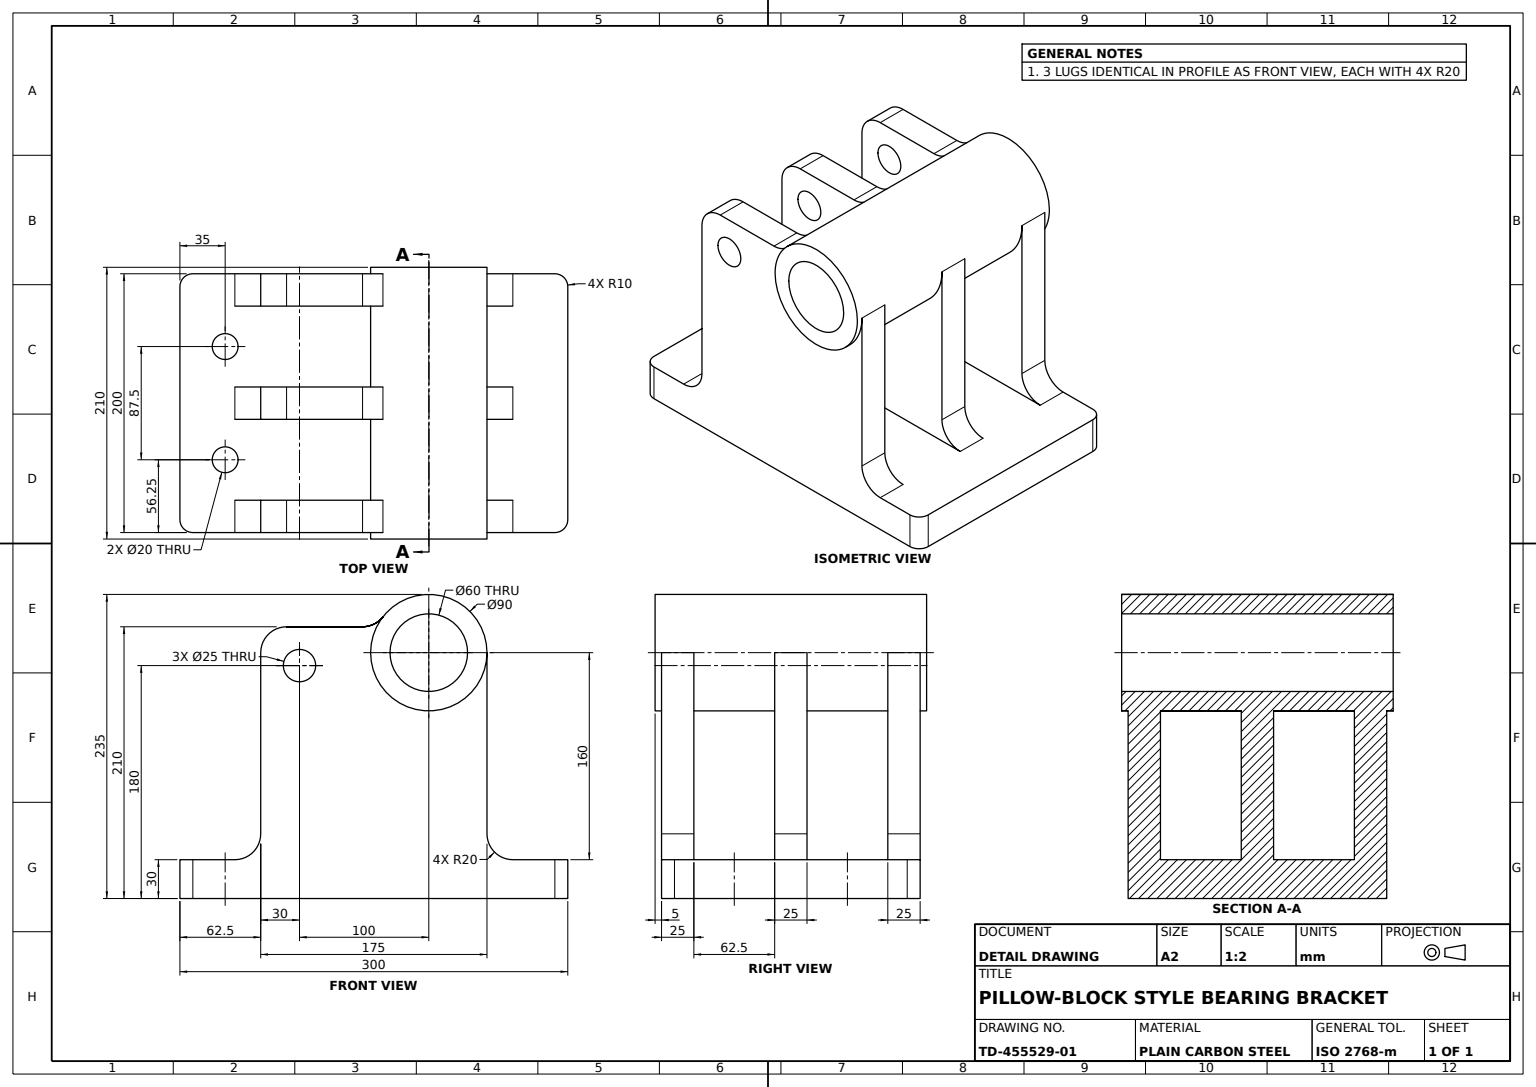
solid
v1 (12.5,50,-87.5)
v2 (-12.5,50,-87.5)
e1 v1 v2 LINE
v3 (12.5,30,-107.5)
e2 v3 v1 CIRCLE(AX(P(12.5,50,-107.5),D(-1,0,0),D(0,0,-1)),20)
v4 (-12.5,30,-107.5)
e3 v4 v3 LINE
e4 v2 v4 CIRCLE(AX(P(-12.5,50,-107.5),D(1,0,0),D(0,0,-1)),20)
face CYL(AX(P(12.5,50,-107.5),D(1,0,0),D(0,0,-1)),20) rev [-e1 -e2 -e3 -e4]
v5 (-75,50,87.5)
v6 (-75,30,107.5)
e5 v5 v6 CIRCLE(AX(P(-75,50,107.5),D(-1,0,0),D(0,0,-1)),20)
v7 (-75,30,-107.5)
e6 v6 v7 LINE
v8 (-75,50,-87.5)
e7 v7 v8 CIRCLE(AX(P(-75,50,-107.5),D(-1,0,0),D(0,0,-1)),20)
v9 (-75,190,-87.5)
e8 v8 v9 LINE
v10 (-75,190,2.5)
e9 v10 v9 CIRCLE(AX(P(-75,190,-42.5),D(1,0,0),D(0,0,-1)),45)
v11 (-75,217.692308,-7.029786)
e10 v11 v10 CIRCLE(AX(P(-75,190,-42.5),D(1,0,0),D(0,0,-1)),45)
v12 (-75,210,8.734754)
e11 v11 v12 CIRCLE(AX(P(-75,230,8.734754),D(-1,0,0),D(0,0,-1)),20)
v13 (-75,210,67.5)
e12 v12 v13 LINE
v14 (-75,190,87.5)
e13 v13 v14 CIRCLE(AX(P(-75,190,67.5),D(1,0,0),D(0,0,-1)),20)
e14 v14 v5 LINE
v15 (-75,180,70)
v16 (-75,180,45)
e15 v15 v16 CIRCLE(AX(P(-75,180,57.5),D(1,0,0),D(0,0,-1)),12.5)
e16 v16 v15 CIRCLE(AX(P(-75,180,57.5),D(1,0,0),D(0,0,-1)),12.5)
face PLANE(AX(P(-75,0,0),D(1,0,0),D(0,0,-1))) [e5 e6 e7 e8 -e9 -e10 e11 e12 e13 e14] [-e15 -e16]
v17 (-12.5,217.692308,-7.029786)
v18 (12.5,217.692308,-7.029786)
e17 v17 v18 LINE
v19 (-12.5,210,8.734754)
e18 v19 v17 CIRCLE(AX(P(-12.5,230,8.734754),D(1,0,0),D(0,0,-1)),20)
v20 (12.5,210,8.734754)
e19 v20 v19 LINE
e20 v18 v20 CIRCLE(AX(P(12.5,230,8.734754),D(-1,0,0),D(0,0,-1)),20)
face CYL(AX(P(-105,230,8.734754),D(1,0,0),D(0,0,-1)),20) rev [-e17 -e18 -e19 -e20]
v21 (-100,180,70)
e21 v21 v15 LINE
v22 (-100,180,45)
e22 v22 v21 CIRCLE(AX(P(-100,180,57.5),D(1,0,0),D(0,0,-1)),12.5)
e23 v22 v16 LINE
face CYL(AX(P(-100,180,57.5),D(1,0,0),D(0,0,-1)),12.5) rev [e16 -e21 -e22 e23]
v23 (-43.75,30,125)
v24 (-43.75,30,105)
e24 v23 v24 CIRCLE(AX(P(-43.75,30,115),D(0,1,0),D(0,0,1)),10)
v25 (-43.75,0,105)
e25 v25 v24 LINE
v26 (-43.75,0,125)
e26 v25 v26 CIRCLE(AX(P(-43.75,0,115),D(0,-1,0),D(0,0,-1)),10)
e27 v26 v23 LINE
face CYL(AX(P(-43.75,-10,115),D(0,1,0),D(0,0,1)),10) rev [e24 -e25 e26 e27]
v27 (43.75,0,105)
v28 (43.75,30,105)
e28 v27 v28 LINE
v29 (43.75,0,125)
e29 v27 v29 CIRCLE(AX(P(43.75,0,115),D(0,-1,0),D(0,0,-1)),10)
v30 (43.75,30,125)
e30 v29 v30 LINE
e31 v30 v28 CIRCLE(AX(P(43.75,30,115),D(0,1,0),D(0,0,1)),10)
face CYL(AX(P(43.75,-10,115),D(0,1,0),D(0,0,1)),10) rev [-e28 e29 e30 e31]
v31 (12.5,190,2.5)
v32 (75,190,2.5)
e32 v31 v32 LINE
v33 (12.5,190,-87.5)
e33 v31 v33 CIRCLE(AX(P(12.5,190,-42.5),D(1,0,0),D(0,0,-1)),45)
v34 (75,190,-87.5)
e34 v33 v34 LINE
e35 v34 v32 CIRCLE(AX(P(75,190,-42.5),D(-1,0,0),D(0,0,1)),45)
face CYL(AX(P(-105,190,-42.5),D(1,0,0),D(0,0,-1)),45) [-e32 e33 e34 e35]
v35 (75,180,45)
v36 (75,180,70)
e36 v35 v36 CIRCLE(AX(P(75,180,57.5),D(-1,0,0),D(0,0,1)),12.5)
e37 v36 v35 CIRCLE(AX(P(75,180,57.5),D(-1,0,0),D(0,0,1)),12.5)
v37 (75,50,-87.5)
e38 v37 v34 LINE
v38 (75,30,-107.5)
e39 v37 v38 CIRCLE(AX(P(75,50,-107.5),D(1,0,0),D(0,0,1)),20)
v39 (75,30,107.5)
e40 v39 v38 LINE
v40 (75,50,87.5)
e41 v39 v40 CIRCLE(AX(P(75,50,107.5),D(1,0,0),D(0,0,1)),20)
v41 (75,190,87.5)
e42 v41 v40 LINE
v42 (75,210,67.5)
e43 v41 v42 CIRCLE(AX(P(75,190,67.5),D(-1,0,0),D(0,0,1)),20)
v43 (75,210,8.734754)
e44 v43 v42 LINE
v44 (75,217.692308,-7.029786)
e45 v43 v44 CIRCLE(AX(P(75,230,8.734754),D(1,0,0),D(0,0,1)),20)
e46 v32 v44 CIRCLE(AX(P(75,190,-42.5),D(-1,0,0),D(0,0,1)),45)
face PLANE(AX(P(75,0,0),D(-1,0,0),D(0,0,1))) [-e36 -e37] [-e38 e39 -e40 e41 -e42 e43 -e44 e45 -e46 -e35]
v45 (100,180,45)
e47 v35 v45 LINE
v46 (100,180,70)
e48 v36 v46 LINE
e49 v46 v45 CIRCLE(AX(P(100,180,57.5),D(1,0,0),D(0,0,-1)),12.5)
face CYL(AX(P(-100,180,57.5),D(1,0,0),D(0,0,-1)),12.5) rev [-e47 e36 e48 e49]
v47 (-100,210,8.734754)
e50 v12 v47 LINE
v48 (-100,210,67.5)
e51 v47 v48 LINE
e52 v48 v13 LINE
face PLANE(AX(P(-65,210,0),D(0,-1,0),D(0,0,-1))) rev [-e12 e50 e51 e52]
v49 (105,190,2.5)
v50 (105,190,-87.5)
e53 v49 v50 CIRCLE(AX(P(105,190,-42.5),D(1,0,0),D(0,0,-1)),45)
v51 (100,190,2.5)
e54 v51 v49 LINE
v52 (100,190,-87.5)
e55 v51 v52 CIRCLE(AX(P(100,190,-42.5),D(1,0,0),D(0,0,-1)),45)
e56 v52 v50 LINE
face CYL(AX(P(-105,190,-42.5),D(1,0,0),D(0,0,-1)),45) [-e53 -e54 e55 e56]
v53 (-100,50,-87.5)
v54 (-100,30,-107.5)
e57 v53 v54 CIRCLE(AX(P(-100,50,-107.5),D(1,0,0),D(0,0,-1)),20)
e58 v8 v53 LINE
e59 v54 v7 LINE
face CYL(AX(P(-65,50,-107.5),D(1,0,0),D(0,0,-1)),20) rev [-e57 -e58 -e7 -e59]
v55 (-100,190,87.5)
e60 v14 v55 LINE
e61 v55 v48 CIRCLE(AX(P(-100,190,67.5),D(-1,0,0),D(0,0,-1)),20)
face CYL(AX(P(-65,190,67.5),D(1,0,0),D(0,0,-1)),20) [-e60 -e13 -e52 -e61]
e62 v21 v22 CIRCLE(AX(P(-100,180,57.5),D(1,0,0),D(0,0,-1)),12.5)
face CYL(AX(P(-100,180,57.5),D(1,0,0),D(0,0,-1)),12.5) rev [e21 e15 -e23 -e62]
e63 v34 v52 LINE
v56 (100,50,-87.5)
e64 v56 v52 LINE
e65 v56 v37 LINE
face PLANE(AX(P(75,30,-87.5),D(0,0,-1),D(-1,0,0))) [e38 e63 -e64 e65]
v57 (-105,190,2.5)
v58 (-100,190,2.5)
e66 v57 v58 LINE
v59 (-105,190,-87.5)
e67 v57 v59 CIRCLE(AX(P(-105,190,-42.5),D(1,0,0),D(0,0,-1)),45)
v60 (-100,190,-87.5)
e68 v59 v60 LINE
e69 v58 v60 CIRCLE(AX(P(-100,190,-42.5),D(1,0,0),D(0,0,-1)),45)
face CYL(AX(P(-105,190,-42.5),D(1,0,0),D(0,0,-1)),45) [-e66 e67 e68 -e69]
e70 v28 v30 CIRCLE(AX(P(43.75,30,115),D(0,1,0),D(0,0,1)),10)
e71 v29 v27 CIRCLE(AX(P(43.75,0,115),D(0,-1,0),D(0,0,-1)),10)
face CYL(AX(P(43.75,-10,115),D(0,1,0),D(0,0,1)),10) rev [e28 e70 -e30 e71]
v61 (-105,190,-72.5)
v62 (-105,190,-12.5)
e72 v61 v62 CIRCLE(AX(P(-105,190,-42.5),D(1,0,0),D(0,0,-1)),30)
e73 v62 v61 CIRCLE(AX(P(-105,190,-42.5),D(1,0,0),D(0,0,-1)),30)
e74 v59 v57 CIRCLE(AX(P(-105,190,-42.5),D(1,0,0),D(0,0,-1)),45)
face PLANE(AX(P(-105,190,-42.5),D(1,0,0),D(0,0,-1))) rev [e72 e73] [-e74 -e67]
e75 v45 v46 CIRCLE(AX(P(100,180,57.5),D(1,0,0),D(0,0,-1)),12.5)
v63 (100,217.692308,-7.029786)
v64 (100,210,8.734754)
e76 v63 v64 CIRCLE(AX(P(100,230,8.734754),D(-1,0,0),D(0,0,1)),20)
v65 (100,210,67.5)
e77 v64 v65 LINE
v66 (100,190,87.5)
e78 v65 v66 CIRCLE(AX(P(100,190,67.5),D(1,0,0),D(0,0,1)),20)
v67 (100,50,87.5)
e79 v66 v67 LINE
v68 (100,30,107.5)
e80 v67 v68 CIRCLE(AX(P(100,50,107.5),D(-1,0,0),D(0,0,1)),20)
v69 (100,30,140)
e81 v69 v68 LINE
v70 (100,0,140)
e82 v69 v70 LINE
v71 (100,0,-140)
e83 v70 v71 LINE
v72 (100,30,-140)
e84 v72 v71 LINE
v73 (100,30,-107.5)
e85 v73 v72 LINE
e86 v73 v56 CIRCLE(AX(P(100,50,-107.5),D(-1,0,0),D(0,0,1)),20)
e87 v63 v51 CIRCLE(AX(P(100,190,-42.5),D(1,0,0),D(0,0,-1)),45)
face PLANE(AX(P(100,30,140),D(-1,0,0),D(0,0,1))) rev [-e75 -e49] [e76 e77 e78 e79 e80 -e81 e82 e83 -e84 -e85 e86 e64 -e55 -e87]
v74 (-100,30,140)
v75 (-100,0,140)
e88 v74 v75 LINE
v76 (-90,0,150)
e89 v75 v76 CIRCLE(AX(P(-90,0,140),D(0,1,0),D(0,0,-1)),10)
v77 (-90,30,150)
e90 v77 v76 LINE
e91 v74 v77 CIRCLE(AX(P(-90,30,140),D(0,1,0),D(0,0,-1)),10)
face CYL(AX(P(-90,30,140),D(0,-1,0),D(0,0,-1)),10) [e88 e89 -e90 -e91]
e92 v18 v31 CIRCLE(AX(P(12.5,190,-42.5),D(1,0,0),D(0,0,-1)),45)
v78 (12.5,210,67.5)
e93 v20 v78 LINE
v79 (12.5,190,87.5)
e94 v78 v79 CIRCLE(AX(P(12.5,190,67.5),D(1,0,0),D(0,0,-1)),20)
v80 (12.5,50,87.5)
e95 v79 v80 LINE
v81 (12.5,30,107.5)
e96 v80 v81 CIRCLE(AX(P(12.5,50,107.5),D(-1,0,0),D(0,0,-1)),20)
e97 v81 v3 LINE
e98 v1 v33 LINE
v82 (12.5,180,70)
v83 (12.5,180,45)
e99 v82 v83 CIRCLE(AX(P(12.5,180,57.5),D(1,0,0),D(0,0,-1)),12.5)
e100 v83 v82 CIRCLE(AX(P(12.5,180,57.5),D(1,0,0),D(0,0,-1)),12.5)
face PLANE(AX(P(12.5,0,0),D(1,0,0),D(0,0,-1))) [-e92 e20 e93 e94 e95 e96 e97 e2 e98 -e33] [-e99 -e100]
v84 (-12.5,30,107.5)
v85 (-12.5,50,87.5)
e101 v84 v85 CIRCLE(AX(P(-12.5,50,107.5),D(1,0,0),D(0,0,-1)),20)
e102 v81 v84 LINE
e103 v85 v80 LINE
face CYL(AX(P(-90,50,107.5),D(1,0,0),D(0,0,-1)),20) rev [-e101 -e102 -e96 -e103]
e104 v68 v39 LINE
e105 v40 v67 LINE
face CYL(AX(P(75,50,107.5),D(1,0,0),D(0,0,-1)),20) rev [-e41 -e104 -e80 -e105]
v86 (-12.5,190,87.5)
v87 (-12.5,210,67.5)
e106 v86 v87 CIRCLE(AX(P(-12.5,190,67.5),D(-1,0,0),D(0,0,-1)),20)
e107 v79 v86 LINE
e108 v87 v78 LINE
face CYL(AX(P(12.5,190,67.5),D(-1,0,0),D(0,0,1)),20) [-e106 -e107 -e94 -e108]
v88 (105,190,-72.5)
e109 v61 v88 LINE
v89 (105,190,-12.5)
e110 v62 v89 LINE
e111 v89 v88 CIRCLE(AX(P(105,190,-42.5),D(1,0,0),D(0,0,-1)),30)
face CYL(AX(P(-105,190,-42.5),D(1,0,0),D(0,0,-1)),30) rev [-e109 -e73 e110 e111]
v90 (90,0,-150)
v91 (-90,0,-150)
e112 v90 v91 LINE
e113 v71 v90 CIRCLE(AX(P(90,0,-140),D(0,1,0),D(0,0,-1)),10)
v92 (90,0,150)
e114 v92 v70 CIRCLE(AX(P(90,0,140),D(0,1,0),D(0,0,1)),10)
e115 v76 v92 LINE
v93 (-100,0,-140)
e116 v93 v75 LINE
e117 v91 v93 CIRCLE(AX(P(-90,0,-140),D(0,1,0),D(0,0,-1)),10)
e118 v26 v25 CIRCLE(AX(P(-43.75,0,115),D(0,-1,0),D(0,0,-1)),10)
face PLANE(AX(P(-90,0,140),D(0,-1,0),D(0,0,-1))) [-e112 -e113 -e83 -e114 -e115 -e89 -e116 -e117] [-e26 -e118] [-e29 -e71]
v94 (-100,50,87.5)
e119 v94 v5 LINE
e120 v94 v55 LINE
face PLANE(AX(P(-65,0,87.5),D(0,0,1),D(1,0,0))) [e119 -e14 e60 -e120]
e121 v38 v73 LINE
face CYL(AX(P(-90,50,-107.5),D(1,0,0),D(0,0,-1)),20) rev [-e65 -e86 -e121 -e39]
e122 v42 v65 LINE
e123 v64 v43 LINE
face PLANE(AX(P(75,210,87.5),D(0,1,0),D(0,0,1))) [e122 -e77 e123 e44]
v95 (90,30,150)
e124 v95 v69 CIRCLE(AX(P(90,30,140),D(0,1,0),D(0,0,1)),10)
e125 v95 v92 LINE
face CYL(AX(P(90,30,140),D(0,-1,0),D(0,0,-1)),10) [-e82 -e124 e125 e114]
v96 (90,30,-150)
e126 v96 v90 LINE
v97 (-90,30,-150)
e127 v97 v91 LINE
e128 v96 v97 LINE
face PLANE(AX(P(-90,30,-150),D(0,0,1),D(1,0,0))) rev [e126 e112 -e127 -e128]
e129 v86 v85 LINE
face PLANE(AX(P(12.5,210,87.5),D(0,0,-1),D(-1,0,0))) rev [e107 e129 e103 -e95]
e130 v88 v89 CIRCLE(AX(P(105,190,-42.5),D(1,0,0),D(0,0,-1)),30)
face CYL(AX(P(-105,190,-42.5),D(1,0,0),D(0,0,-1)),30) rev [e130 -e110 -e72 e109]
e131 v44 v63 LINE
face CYL(AX(P(-105,230,8.734754),D(1,0,0),D(0,0,-1)),20) rev [-e131 -e45 -e123 -e76]
e132 v84 v4 LINE
e133 v19 v87 LINE
v98 (-12.5,190,2.5)
e134 v17 v98 CIRCLE(AX(P(-12.5,190,-42.5),D(1,0,0),D(0,0,-1)),45)
v99 (-12.5,190,-87.5)
e135 v98 v99 CIRCLE(AX(P(-12.5,190,-42.5),D(1,0,0),D(0,0,-1)),45)
e136 v2 v99 LINE
v100 (-12.5,180,45)
v101 (-12.5,180,70)
e137 v100 v101 CIRCLE(AX(P(-12.5,180,57.5),D(1,0,0),D(0,0,-1)),12.5)
e138 v101 v100 CIRCLE(AX(P(-12.5,180,57.5),D(1,0,0),D(0,0,-1)),12.5)
face PLANE(AX(P(-12.5,0,0),D(1,0,0),D(0,0,-1))) rev [-e132 e101 -e129 e106 -e133 e18 e134 e135 -e136 e4] [e137 e138]
e139 v100 v83 LINE
e140 v101 v82 LINE
face CYL(AX(P(-100,180,57.5),D(1,0,0),D(0,0,-1)),12.5) rev [-e139 -e138 e140 e99]
face CYL(AX(P(-100,180,57.5),D(1,0,0),D(0,0,-1)),12.5) rev [e100 -e140 -e137 e139]
e141 v50 v49 CIRCLE(AX(P(105,190,-42.5),D(1,0,0),D(0,0,-1)),45)
face PLANE(AX(P(105,190,-42.5),D(1,0,0),D(0,0,-1))) [-e130 -e111] [e141 e53]
e142 v66 v41 LINE
face CYL(AX(P(75,190,67.5),D(1,0,0),D(0,0,-1)),20) [-e43 -e142 -e78 -e122]
e143 v53 v60 LINE
v102 (-100,30,-140)
e144 v102 v54 LINE
e145 v102 v93 LINE
v103 (-100,30,107.5)
e146 v103 v74 LINE
e147 v103 v94 CIRCLE(AX(P(-100,50,107.5),D(1,0,0),D(0,0,-1)),20)
v104 (-100,217.692308,-7.029786)
e148 v47 v104 CIRCLE(AX(P(-100,230,8.734754),D(1,0,0),D(0,0,-1)),20)
e149 v104 v58 CIRCLE(AX(P(-100,190,-42.5),D(1,0,0),D(0,0,-1)),45)
face PLANE(AX(P(-100,30,140),D(1,0,0),D(0,0,-1))) rev [-e143 e57 -e144 e145 e116 -e88 -e146 e147 e120 e61 -e51 e148 e149 e69] [e22 e62]
e150 v99 v33 LINE
face PLANE(AX(P(12.5,30,-87.5),D(0,0,1),D(1,0,0))) rev [e1 e136 e150 -e98]
e151 v72 v96 CIRCLE(AX(P(90,30,-140),D(0,1,0),D(0,0,-1)),10)
face CYL(AX(P(90,30,-140),D(0,-1,0),D(0,0,-1)),10) [-e151 e84 e113 -e126]
face PLANE(AX(P(12.5,210,-87.5),D(0,-1,0),D(0,0,-1))) rev [-e93 e19 e133 e108]
face CYL(AX(P(-100,180,57.5),D(1,0,0),D(0,0,-1)),12.5) rev [-e48 e37 e47 e75]
e152 v10 v98 LINE
e153 v9 v99 LINE
face CYL(AX(P(-105,190,-42.5),D(1,0,0),D(0,0,-1)),45) [-e135 -e152 e9 e153]
e154 v60 v9 LINE
e155 v104 v11 LINE
face CYL(AX(P(-105,190,-42.5),D(1,0,0),D(0,0,-1)),45) [-e153 -e154 -e68 e74 e66 -e149 e155 e10 e152 -e134 e17 e92 e32 e46 e131 e87 e54 -e141 -e56 -e63 -e34 -e150]
face CYL(AX(P(-105,230,8.734754),D(1,0,0),D(0,0,-1)),20) rev [-e155 -e148 -e50 -e11]
e156 v97 v102 CIRCLE(AX(P(-90,30,-140),D(0,1,0),D(0,0,-1)),10)
face CYL(AX(P(-90,30,-140),D(0,-1,0),D(0,0,-1)),10) [-e145 -e156 e127 e117]
e157 v24 v23 CIRCLE(AX(P(-43.75,30,115),D(0,1,0),D(0,0,1)),10)
face CYL(AX(P(-43.75,-10,115),D(0,1,0),D(0,0,1)),10) rev [e157 -e27 e118 e25]
face PLANE(AX(P(75,30,87.5),D(0,0,1),D(1,0,0))) [e142 e42 e105 -e79]
e158 v6 v103 LINE
face CYL(AX(P(-90,50,107.5),D(-1,0,0),D(0,0,1)),20) rev [-e158 -e5 -e119 -e147]
face PLANE(AX(P(-65,0,-87.5),D(0,0,1),D(1,0,0))) rev [e154 -e8 e58 e143]
e159 v77 v95 LINE
face PLANE(AX(P(-90,30,140),D(0,-1,0),D(0,0,-1))) rev [e159 e124 e81 e104 e40 e121 e85 e151 e128 e156 e144 e59 -e6 e158 e146 e91] [-e97 e102 e132 e3] [-e157 -e24] [-e31 -e70]
face PLANE(AX(P(-90,30,150),D(0,0,-1),D(-1,0,0))) rev [e115 -e125 -e159 e90]
